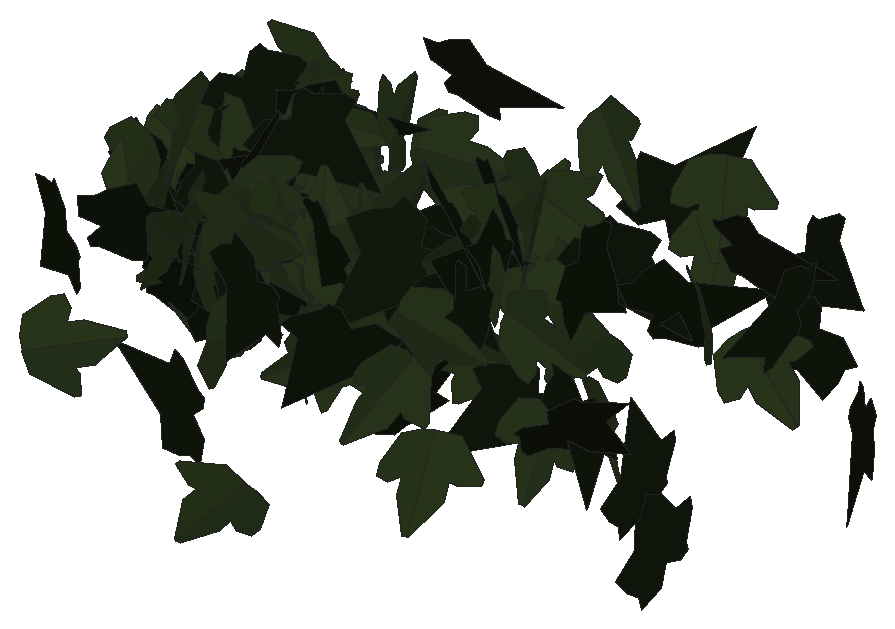
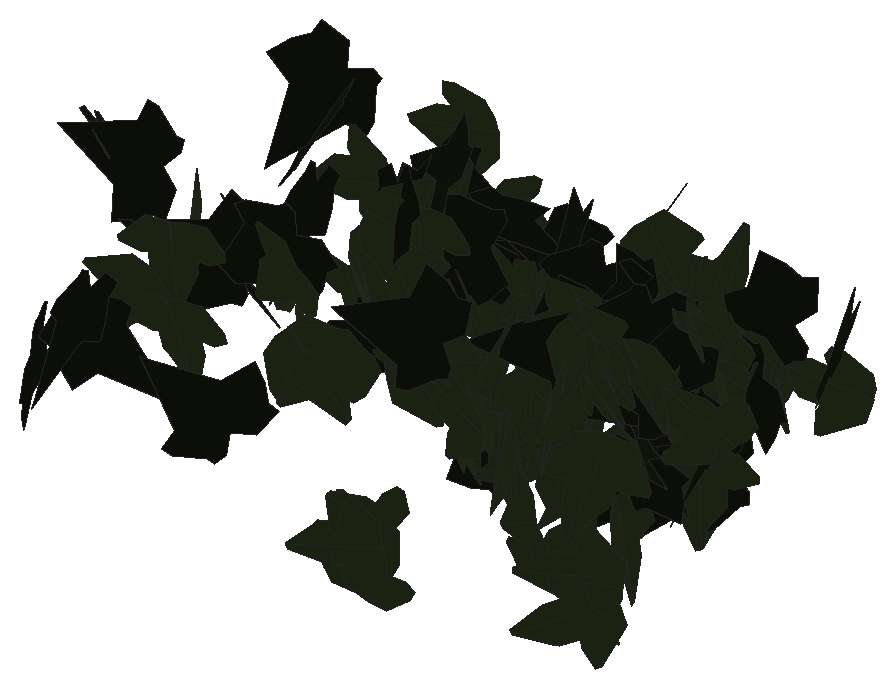
# SketchUp Ruby script. Lengths in inches.
U = 1.inch
M = Sketchup.active_model
def pt(a) = Geom::Point3d.new(a.map { |v| v * U })
def face(e, loops, mat)
  f = e.add_face(loops[0].map { |a| pt(a) })
  loops[1..].each { |l| e.add_face(l.map { |a| pt(a) }).erase! }
  f.material = f.back_material = mat if mat
  f
end
# faces: each face lists its corners as indices into pts; further lists are holes
def faces(e, pts, list, mat = nil) = list.each { |f| face(e, (f[0].is_a?(Array) ? f : [f]).map { |l| l.map { |i| pts[i] } }, mat) }
# xy, xz, yz: faces in a plane at the given z, y or x. An outline is a flat list of corners, or four numbers for a rectangle; further outlines are holes
def ring(l) = l.size == 4 ? [[l[0], l[1]], [l[2], l[1]], [l[2], l[3]], [l[0], l[3]]] : l.each_slice(2).to_a
def flat(e, list, mat, &to3) = list.each { |f| face(e, (f[0].is_a?(Array) ? f : [f]).map { |l| ring(l).map { |u, v| to3.(u, v) } }, mat) }
def xy(e, z, list, mat = nil) = flat(e, list, mat) { |x, y| [x, y, z] }
def xz(e, y, list, mat = nil) = flat(e, list, mat) { |x, z| [x, y, z] }
def yz(e, x, list, mat = nil) = flat(e, list, mat) { |y, z| [x, y, z] }
def lines(e, pts, list) = list.each { |a, b| e.add_line(pt(pts[a]), pt(pts[b])) }
# prism: a flat outline (further loops are holes) pulled along v
def prism(e, loops, v, mat = nil)
  f = face(e, loops, mat); d = Geom::Vector3d.new(v.map { |x| x * U })
  f.pushpull(f.normal.samedirection?(d) ? d.length : -d.length)
end
def box(e, o, s, mat = nil) = prism(e, [[o, [o[0] + s[0], o[1], o[2]], [o[0] + s[0], o[1] + s[1], o[2]], [o[0], o[1] + s[1], o[2]]]], [0, 0, s[2]], mat)
def at(x, y, z, deg = 0) = Geom::Transformation.translation(pt([x, y, z])) * Geom::Transformation.rotation(ORIGIN, Z_AXIS, deg.degrees)
def axes(o, x, y, z) = Geom::Transformation.new([*x, 0, *y, 0, *z, 0, *pt(o).to_a, 1])
def part(name) = M.definitions.add(name)
# library, detail: a bought-in or finely detailed component or shape, given as its bounding box
def library(name, o, s) = part(name).tap { |d| box(d.entities, o, s) }
def detail(e, o, s) = box(e.add_group.entities, o, s)
def put(e, d, t, mat = nil) = e.add_instance(d, t).tap { |i| i.material = mat if mat }
def group(e, t, mat = nil) = e.add_group.tap { |g| g.transformation = t; g.material = mat if mat }.entities
root = M.entities
M.materials.add("efeu1").color = [18, 25, 13]
M.materials.add("efeu2").color = [43, 57, 29]
c1 = part("ivyleaf_9")
p = [[1.54,2.16,1.25],[1.36,2.04,1.19],[-0.21,0.99,0.68],[-0.71,1.11,0.82],[-0.85,0.86,0.67],[-0.8,0.17,0.21],
  [-0.9,-0.01,0.1],[-0.67,-0.16,-0.02],[-0.08,-0.08,-0.05],[-0.03,-0.6,-0.4],[0.65,-0.88,-0.66],[0.83,-0.6,-0.49],
  [1.29,-0.42,-0.43],[1.8125,-0.07,-0.26],[1.21,0.44,0.15]]
faces(c1.entities,p,[[0,1,2,3,4,5,6,7,8,9,10,11,12,13,14]],"efeu1")
c2 = part("ivyleaf_10")
p = [[0,0.5,-0.03],[-0.0625,2.02,-0.43],[-0.19,2.01,-0.46],[-0.54,1.05,-0.29],[-0.52,0.625,-0.18],[-0.83,0.76,-0.28],
  [-1.16,0.64,-0.33],[-1.15,0.33,-0.24],[-0.77,-0.39,0.02],[-0.3,-0.51,0.16],[0.04,-0.48,0.23],[-0.02,2.01,-0.4375],
  [-0.06,2.01,-0.43],[0.04,-0.49,0.23],[0.67,-0.49,0.14],[1.38,0.36,-0.2],[1.375,0.51,-0.24],[0.81,0.65,-0.19],
  [0.62,0.59,-0.15],[0.6,1.09,-0.28],[0.5,1.23,-0.31]]
faces(c2.entities,p,[[0,1,2,3,4,5,6,7,8,9,10],[11,12,0,13,14,15,16,17,18,19,20]],"efeu2")
put(root,c1,axes([25.31,222.52,197.26],[-0.0221,-0.19692,0.45906],[0.03288,-0.45908,-0.19535],[0.49843,0.02155,0.03324]))
put(root,c2,axes([25.57,223.58,197.92],[0.40986,-0.22093,-0.18221],[-0.16013,0.08695,-0.46562],[0.23743,0.44003,0.00052]))
put(root,c2,axes([25.3,224.54,197.3],[0.31203,0.19851,-0.3365],[0.27533,0.19381,0.36964],[0.27719,-0.41597,0.01163]))
put(root,c2,axes([25.28,226.79,196.36],[-0.05443,-0.02916,0.49617],[0.37588,0.32415,0.06029],[-0.32519,0.37957,-0.01336]))
put(root,c2,axes([25.33,226.82,196.02],[-0.16477,-0.09139,-0.46314],[0.42786,0.17836,-0.18742],[0.19947,-0.45808,0.01943]))
put(root,c1,axes([25.29,223.83,197.75],[-0.03451,-0.02674,-0.49809],[0.48073,0.13142,-0.04036],[0.13308,-0.48168,0.01664]))
put(root,c2,axes([25.67,226.31,197.6875],[-0.36185,-0.29618,-0.17704],[0.1368,0.11237,-0.46761],[0.31678,-0.38684,-0.00029]))
put(root,c2,axes([25.44,223.65,197.35],[0.27571,0.12766,-0.3971],[0.3444,0.19887,0.30305],[0.23532,-0.44063,0.02173]))
put(root,c1,axes([25.64,224.06,197.17],[0.35436,-0.23145,-0.26619],[-0.22196,0.14695,-0.42325],[0.27415,0.41814,0.0014]))
put(root,c2,axes([25.92,223.7,197.8],[0.16695,-0.46957,0.04035],[0.01767,-0.03654,-0.49835],[0.47097,0.16783,0.0044]))
put(root,c2,axes([25.99,225.99,196.0625],[0.3583,-0.32827,-0.11771],[-0.08261,0.08407,-0.48591],[0.33882,0.36765,0.00601]))
put(root,c2,axes([26.1,223.98,196.41],[-0.3707,-0.33432,0.02854],[-0.02074,-0.01961,-0.49918],[0.3349,-0.37127,0.00067]))
put(root,c2,axes([25.75,223.875,198.11],[0.23673,0.10076,0.42873],[0.38985,0.1785,-0.25721],[-0.20489,0.45605,0.00595]))
put(root,c2,axes([26,224.08,198.53],[0.13252,-0.30003,0.37738],[0.17175,-0.33633,-0.3277],[0.45049,0.21648,0.01392]))
put(root,c2,axes([26.01,224.48,197.47],[0.08977,-0.24396,0.42711],[0.24999,-0.35128,-0.25319],[0.42361,0.259,0.05891]))
put(root,c2,axes([25.81,221.52,196.37],[0.12709,0.01339,-0.48339],[0.47817,0.07107,0.12769],[0.07213,-0.49474,0.00526]))
put(root,c2,axes([26.23,224.96,198.22],[0.47878,-0.10118,-0.10263],[-0.10059,0.0204,-0.48935],[0.10321,0.48923,-0.00082]))
put(root,c2,axes([26.13,224.24,198.35],[0.49854,0.02907,0.02481],[0.02477,0.00136,-0.49938],[-0.0291,0.49915,-0.00008]))
put(root,c1,axes([25.88,223.68,196.25],[0.40019,-0.04094,0.29694],[0.29495,-0.03456,-0.40226],[0.05346,0.49712,-0.00351]))
put(root,c2,axes([26.6,225.54,198.6],[-0.32265,-0.0778,0.37396],[-0.34779,-0.14255,-0.32973],[0.15792,-0.47289,0.03787]))
put(root,c1,axes([25.92,224.45,197.66],[0.22301,-0.00478,0.44749],[0.44718,0.02158,-0.22263],[-0.01718,0.49951,0.01391]))
put(root,c1,axes([26.57,224.21,196.51],[-0.35904,0.1823,-0.29641],[-0.26477,0.13324,0.40267],[0.2258,0.44611,0.00086]))
put(root,c1,axes([26.02,223.78,197.21],[0.00992,-0.03522,-0.49866],[0.24826,0.43325,-0.02566],[0.4339,-0.24709,0.02608]))
put(root,c2,axes([26.61,225.47,198.21],[0.16874,-0.11481,-0.45645],[-0.37332,0.26265,-0.20407],[0.28664,0.40967,0.00292]))
put(root,c2,axes([26.37,225.02,196.06],[0.13316,-0.47667,-0.07111],[-0.0116,0.07058,-0.49486],[0.4818,0.13344,0.00773]))
put(root,c1,axes([25.99,222.4375,197.61],[0.27317,0.03056,0.41766],[0.41302,0.06276,-0.27473],[-0.06922,0.4951,0.00904]))
put(root,c1,axes([26.13,223.99,197.4375],[0.33864,0.13861,0.34075],[0.31226,0.13651,-0.36586],[-0.19446,0.4606,0.00589]))
put(root,c1,axes([26.31,224.61,198.68],[0.02579,-0.243,-0.43622],[-0.02738,0.43545,-0.24419],[0.49858,0.03648,0.00915]))
put(root,c1,axes([26.33,224.8,196.6875],[-0.15803,-0.18918,-0.43502],[0.2796,0.33326,-0.2465],[0.38321,-0.32117,0.00046]))
put(root,c2,axes([26.64,225.51,197.88],[0.02106,-0.10298,-0.48883],[0.01306,0.48921,-0.10249],[0.49939,-0.00845,0.0233]))
put(root,c2,axes([26.33,226.73,196.76],[0.20715,-0.07478,0.44888],[0.43504,-0.11215,-0.21945],[0.13351,0.48149,0.0186]))
put(root,c1,axes([26.85,223.84,196.59],[-0.07456,-0.48679,0.08649],[0.01306,0.0855,0.49246],[-0.49424,0.07569,-0.00004]))
put(root,c2,axes([26.83,225.64,197.9],[-0.25746,0.28819,0.31727],[-0.21018,0.23767,-0.38645],[-0.37355,-0.33235,-0.00124]))
put(root,c1,axes([26.61,223.74,195.86],[0.0041,0.02349,0.49943],[0.34103,0.3651,-0.01997],[-0.36562,0.34081,-0.01303]))
put(root,c2,axes([26.84,225.65,195.48],[0.37583,0.27118,0.18765],[-0.15597,-0.1045,0.46341],[0.29056,-0.40687,0.00604]))
put(root,c1,axes([27.07,224.66,197.97],[-0.04143,0.17819,0.46533],[-0.15839,0.43801,-0.18183],[-0.47244,-0.16247,0.02015]))
put(root,c2,axes([27.13,224.33,196.32],[-0.36002,0.02639,0.34596],[-0.34628,0.00391,-0.36066],[-0.02174,-0.49929,0.01546]))
put(root,c2,axes([26.86,222.63,197.62],[-0.0711,-0.34168,-0.35805],[-0.02501,-0.35878,0.34735],[-0.49429,0.0673,0.03393]))
put(root,c2,axes([26.71,223.2,197.81],[0.1754,-0.1994,0.42365],[0.27895,-0.31885,-0.26556],[0.37606,0.32951,-0.00061]))
put(root,c2,axes([26.88,224.77,196.45],[-0.01878,0.21415,0.45143],[-0.01247,0.45141,-0.21465],[-0.49949,-0.01932,-0.01162]))
put(root,c1,axes([26.5625,223.92,196.42],[0.40028,-0.00746,0.29953],[0.29959,0.0024,-0.4003],[0.00454,0.49994,0.0064]))
put(root,c2,axes([27.16,222.76,197.29],[-0.10793,0.10627,0.47651],[-0.30941,0.3626,-0.15095],[-0.37764,-0.32746,-0.01251]))
put(root,c1,axes([27.07,222.61,195.44],[0.09645,-0.48923,0.03682],[0.00271,0.03806,0.49854],[-0.4906,-0.09597,0.00999]))
put(root,c1,axes([26.85,223.61,197.85],[0.02276,-0.48548,0.11745],[0.00598,-0.1173,-0.48601],[0.49945,0.02353,0.00047]))
put(root,c1,axes([27,223.81,198.05],[0.09998,0.13685,0.4704],[0.15556,0.44638,-0.16293],[-0.46455,0.17893,0.04668]))
put(root,c1,axes([26.83,225.03,198.14],[0.28775,0.03663,0.40726],[0.40514,0.04185,-0.29002],[-0.05533,0.4969,-0.0056]))
put(root,c2,axes([27.02,224.9,198.34],[0.10921,0.11067,0.47521],[0.27526,0.3881,-0.15364],[-0.40287,0.29518,0.02385]))
put(root,c2,axes([27.43,225.82,197.11],[0.07633,-0.2621,-0.4189],[-0.08506,0.41057,-0.27239],[0.48676,0.11285,0.01808]))
put(root,c2,axes([27.22,223.52,198.07],[-0.237,-0.22772,-0.37679],[0.28088,0.25131,-0.32856],[0.33902,-0.3674,0.0088]))
put(root,c2,axes([27.53,224.37,196.9],[0.23081,-0.3063,-0.3208],[-0.18325,0.26347,-0.38341],[0.40392,0.29456,0.00936]))
put(root,c2,axes([27.16,223.74,197.86],[0.38825,-0.11178,0.29457],[0.28256,-0.08324,-0.40402],[0.13936,0.48018,-0.00147]))
put(root,c1,axes([27.33,224.21,198.65],[-0.00303,-0.14018,-0.47994],[0.02025,0.47952,-0.14018],[0.49958,-0.02028,0.00277]))
put(root,c2,axes([27.36,224.21,197],[-0.42033,-0.05443,0.26526],[0.26629,0.00574,0.42315],[-0.04911,0.497,0.02416]))
put(root,c2,axes([27.84,222.62,198.14],[-0.37333,-0.09067,0.32001],[-0.3111,-0.07498,-0.38418],[0.11765,-0.48596,-0.00043]))
put(root,c2,axes([27.31,223.52,197.39],[-0.28358,-0.00816,0.41172],[0.41075,-0.04129,0.2821],[0.02939,0.49823,0.03012]))
put(root,c2,axes([27.7,225.54,198.07],[0.03868,0.1055,-0.48721],[-0.07722,0.48404,0.09868],[0.49249,0.06761,0.05373]))
put(root,c2,axes([27.47,224.88,196.54],[-0.02023,-0.09579,-0.49032],[0.31622,0.37745,-0.08679],[0.38677,-0.31361,0.04531]))
put(root,c2,axes([27.64,222.41,196.74],[-0.02674,-0.15265,-0.47538],[0.12603,0.45858,-0.15434],[0.48312,-0.12808,0.01396]))
put(root,c2,axes([27.35,223.49,197.71],[0.00413,0.00127,-0.49998],[0.42141,-0.26908,0.0028],[-0.26906,-0.42142,-0.00329]))
put(root,c2,axes([27.74,224.8125,197.43],[-0.00165,-0.04137,-0.49828],[0.12552,0.48229,-0.04046],[0.48398,-0.12523,0.00879]))
put(root,c2,axes([27.87,225.25,196.97],[-0.32196,-0.38225,0.01504],[-0.00231,-0.01771,-0.49968],[0.38254,-0.32182,0.00964]))
put(root,c2,axes([27.63,226.3,197.42],[0.10355,-0.07355,-0.4836],[0.41778,-0.24382,0.12653],[-0.25443,-0.43028,0.01096]))
put(root,c2,axes([27.96,223.95,197.29],[0.49415,0.07189,0.02552],[-0.02526,-0.00366,0.49935],[0.07198,-0.49479,0.00002]))
put(root,c2,axes([27.96,225.625,197.39],[0.11434,-0.34982,0.33845],[0.10071,-0.32314,-0.36802],[0.47622,0.15233,-0.00344]))
put(root,c2,axes([28.28,223.78,196.17],[0.01796,0.01815,-0.49935],[-0.24357,-0.43597,-0.02461],[-0.43629,0.24413,-0.00682]))
put(root,c2,axes([27.92,223.59,196.24],[-0.04872,0.04445,-0.49563],[0.26919,-0.41649,-0.06381],[-0.41853,-0.27305,0.01665]))
put(root,c2,axes([28.43,227.22,195.45],[0.4224,0.17373,0.20345],[-0.18911,-0.07508,0.45673],[0.18925,-0.4628,0.00228]))
put(root,c1,axes([27.91,226.49,198.49],[0.27142,-0.1083,0.40571],[0.38604,-0.12574,-0.29182],[0.16524,0.47166,0.01536]))
put(root,c2,axes([28.29,227.18,196.18],[0.20065,0.29652,-0.34902],[0.17098,0.30499,0.35741],[0.42486,-0.26278,0.021]))
put(root,c1,axes([28.31,222.28,197.73],[-0.02242,-0.36861,0.33708],[0.01137,-0.33771,-0.36854],[0.49937,-0.00886,0.02353]))
put(root,c2,axes([28.29,223.38,196.32],[-0.06401,-0.17425,0.46426],[0.17,0.43204,0.1856],[-0.46584,0.18161,0.00393]))
put(root,c2,axes([28.1,227.62,196.21],[0.08919,0.01161,0.49184],[0.44885,0.20275,-0.08618],[-0.20144,0.4569,0.02574]))
put(root,c2,axes([28.16,225.85,197.85],[-0.07424,-0.02934,-0.49359],[0.49389,0.01959,-0.07545],[0.02377,-0.49875,0.02607]))
put(root,c2,axes([28.26,223.63,197.38],[0.07138,0.00742,0.49482],[0.42983,0.24684,-0.0657],[-0.24525,0.43476,0.02886]))
put(root,c2,axes([28.43,223.97,196.17],[0.00766,-0.00567,0.49991],[0.37839,0.32683,-0.00209],[-0.32674,0.37835,0.0093]))
put(root,c2,axes([28.88,223.72,197.46],[0.40405,-0.12717,0.26565],[-0.25288,0.08137,0.42359],[-0.15097,-0.47666,0.00144]))
put(root,c1,axes([28.54,223.37,197.96],[0.2874,-0.16874,-0.37273],[0.32392,-0.18443,0.33326],[-0.24995,-0.43303,0.0033]))
put(root,c2,axes([28.91,224.87,196.45],[0.21003,-0.42996,0.14498],[0.07228,-0.12602,-0.47843],[0.44795,0.22193,0.00922]))
put(root,c2,axes([29.12,223.93,196.98],[-0.00911,0.3924,0.30974],[-0.01378,-0.30987,0.39216],[0.49973,-0.00139,0.01646]))
put(root,c2,axes([29.41,220.49,196.13],[-0.30694,-0.19223,0.34473],[-0.27983,-0.202,-0.36179],[0.27836,-0.41502,0.01642]))
put(root,c1,axes([29.01,223.81,195.54],[0.18215,0.46441,-0.03387],[-0.00682,0.03903,0.49843],[0.46559,-0.18112,0.02055]))
put(root,c1,axes([29.6,222.375,197.5],[0.11709,0.21514,-0.4359],[-0.20486,-0.38476,-0.24493],[-0.44082,0.23595,-0.00196]))
put(root,c2,axes([29.55,225.03,198.07],[0.04863,-0.48945,0.08987],[0.01094,-0.08923,-0.49185],[0.49751,0.0498,0.00203]))
put(root,c1,axes([29.8,223.37,198.22],[-0.45629,-0.18178,0.09359],[-0.08701,-0.03449,-0.49116],[0.18502,-0.46451,-0.00016]))
put(root,c2,axes([30.03,224.37,196.4],[-0.11783,0.02242,-0.4854],[-0.47329,-0.11842,0.10942],[-0.11006,0.48526,0.04913]))
put(root,c2,axes([29.84,225.375,198.2],[0.32633,-0.27954,-0.25566],[-0.1841,0.17789,-0.42949],[0.33108,0.37445,0.01318]))
put(root,c1,axes([29.4375,223.65,198],[0.16089,0.12233,-0.45733],[0.16175,0.43974,0.17453],[0.44492,-0.20411,0.10193]))
put(root,c2,axes([29.54,226.125,197.53],[0.22057,0.20207,0.40064],[0.2657,0.30093,-0.29806],[-0.36159,0.34439,0.02537]))
put(root,c2,axes([29.64,223.77,196.98],[0.44202,-0.1767,-0.15297],[0.14177,-0.05745,0.47603],[-0.1858,-0.46419,-0.00068]))
put(root,c2,axes([29.85,223.8,197.44],[-0.31435,-0.36726,-0.12769],[0.078,0.1013,-0.48338],[0.38092,-0.32382,-0.00639]))
put(root,c1,axes([29.62,223.65,197.92],[-0.08019,-0.14594,-0.47146],[0.23874,0.40656,-0.16646],[0.43194,-0.25181,0.00448]))
put(root,c2,axes([29.93,224.29,198.41],[0.49014,0.08621,0.04831],[0.04704,0.01145,-0.49765],[-0.08692,0.49238,0.00311]))
put(root,c1,axes([30.29,224.28,198.7],[0.24082,0.00846,-0.4381],[-0.43817,0.00109,-0.24084],[-0.00313,0.49993,0.00794]))
put(root,c2,axes([30.25,224.55,198.4],[-0.0719,-0.2966,0.39605],[-0.07962,-0.38806,-0.30507],[0.48836,-0.10693,0.00857]))
put(root,c2,axes([30.09,223.83,198.03],[-0.04243,-0.19098,-0.46014],[-0.01494,-0.46111,0.19276],[-0.49797,0.03011,0.03342]))
put(root,c2,axes([30.1,225.24,198.14],[0.28531,-0.31459,0.26387],[0.17888,-0.194,-0.4247],[0.36959,0.33675,0.00185]))
put(root,c1,axes([29.93,223.82,198.66],[0.20041,-0.3289,0.31884],[0.15001,-0.2817,-0.38489],[0.43282,0.24993,-0.01423]))
put(root,c1,axes([30.19,227.54,196.99],[-0.11584,-0.06209,0.48242],[0.46946,0.11545,0.12759],[-0.12723,0.48251,0.03155]))
put(root,c2,axes([30.14,226.41,198.6],[0.33247,-0.0094,0.37333],[0.37279,-0.02149,-0.33252],[0.0223,0.49945,-0.00728]))
put(root,c2,axes([30.55,222.14,197.36],[0.17669,0.27835,-0.3759],[-0.19823,-0.31939,-0.32969],[-0.42366,0.26553,-0.00251]))
put(root,c2,axes([30.56,223.73,198.0625],[0.41259,-0.2565,-0.11822],[-0.10133,0.06092,-0.48582],[0.26363,0.42485,-0.00171]))
put(root,c1,axes([30.58,223.72,197.89],[0.02389,0.0358,0.49814],[-0.22947,-0.44217,0.04278],[0.44359,-0.23066,-0.00469]))
put(root,c1,axes([30.68,223.13,198.03],[-0.01143,0.00556,-0.49984],[0.17168,-0.46951,-0.00915],[-0.46946,-0.17183,0.00883]))
put(root,c2,axes([31.07,225.13,196.7],[-0.32933,-0.14778,0.34598],[-0.3167,-0.13932,-0.36096],[0.20309,-0.45689,-0.00184]))
put(root,c1,axes([31.08,223.95,196.49],[0.01439,0.03814,-0.49834],[-0.18737,-0.46177,-0.04075],[-0.46334,0.18792,0.001]))
put(root,c2,axes([31.04,222.0625,196.55],[0.31996,0.36103,-0.13146],[-0.09079,-0.09519,-0.48239],[-0.37334,0.33256,0.00464]))
put(root,c2,axes([30.92,222.01,198.27],[-0.11852,0.04202,-0.48393],[0.47213,-0.10715,-0.12494],[-0.11421,-0.48657,-0.01428]))
put(root,c1,axes([31.54,224.23,198.27],[0.10866,-0.13028,-0.47034],[-0.32987,0.33553,-0.16914],[0.3597,0.34706,-0.01303]))
put(root,c1,axes([31.26,224.99,198.03],[-0.03938,-0.08175,-0.4917],[0.33577,0.36018,-0.08677],[0.36839,-0.33703,0.02653]))
put(root,c2,axes([31.65,226.66,197.6],[0.49602,0.04789,-0.04086],[-0.04063,-0.0043,-0.49833],[-0.04808,0.49768,-0.00037]))
put(root,c2,axes([31.68,223.32,196.58],[0.49405,-0.07503,-0.01686],[-0.01638,0.00441,-0.49971],[0.07514,0.49432,0.0019]))
put(root,c2,axes([31.48,223.18,197.88],[0.11734,0.00725,0.48598],[0.47502,0.10415,-0.11625],[-0.10292,0.48898,0.01755]))
put(root,c2,axes([31.82,226.49,198.51],[0.46635,0.17911,0.02083],[0.01939,0.00761,-0.49957],[-0.17927,0.46676,0.00015]))
put(root,c2,axes([32.09,223.8,196.86],[-0.32016,0.28573,-0.25662],[0.18243,-0.18085,-0.42897],[-0.33796,-0.36831,0.01155]))
put(root,c1,axes([32.01,225.08,197.41],[0.14398,-0.02988,0.47789],[0.4788,0.01406,-0.14337],[-0.00487,0.49891,0.03266]))
put(root,c2,axes([32.6,225.2,197.38],[-0.33293,0.25908,0.26839],[0.2134,-0.16279,0.42185],[0.30597,0.39545,-0.00218]))
put(root,c1,axes([32.73,226.93,197.62],[0.11423,-0.15247,-0.46228],[-0.28045,0.3675,-0.19051],[0.39787,0.30282,-0.00156]))
put(root,c1,axes([33.15,226.54,196.94],[-0.02426,0.06278,-0.49545],[-0.36882,-0.3367,-0.0246],[-0.33673,0.36427,0.06264]))
put(root,c1,axes([33.43,223.05,196.45],[-0.39298,0.12565,-0.28245],[-0.26798,0.08927,0.41257],[0.1541,0.47565,-0.00282]))
put(root,c1,axes([32.93,222.51,197.64],[0.10366,-0.43751,0.21873],[0.04837,-0.21332,-0.44961],[0.48674,0.11438,-0.0019]))
put(root,c2,axes([33.03,225.51,197.06],[0.34203,0.23499,0.27892],[0.21607,0.1775,-0.4145],[-0.29382,0.40407,0.01987]))
put(root,c1,axes([32.97,225.32,198.52],[0.27771,0.132,-0.39427],[0.353,0.17567,0.30746],[0.21969,-0.44913,0.00438]))
put(root,c1,axes([33.3125,221.49,197.97],[0.32454,0.35835,0.12752],[0.08186,0.09789,-0.48344],[-0.37145,0.33467,0.00487]))
put(root,c1,axes([33.88,222.84,195.8],[-0.3936,0.08358,-0.29681],[-0.28973,0.06447,0.40237],[0.10553,0.48873,-0.00232]))
put(root,c1,axes([34.24,224.77,198.33],[-0.38972,0.30928,0.04964],[-0.04134,0.02777,-0.49751],[-0.3105,-0.39188,0.00393]))
put(root,c1,axes([33.95,226.43,196.15],[-0.01445,0.00378,-0.49978],[0.43425,-0.24742,-0.01443],[-0.24742,-0.43447,0.00387]))
